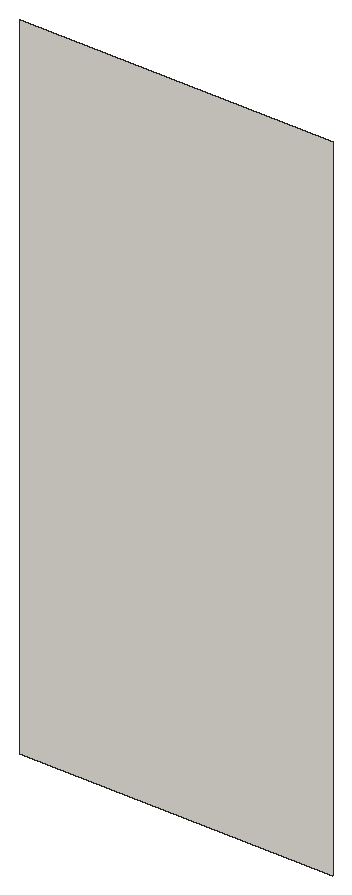
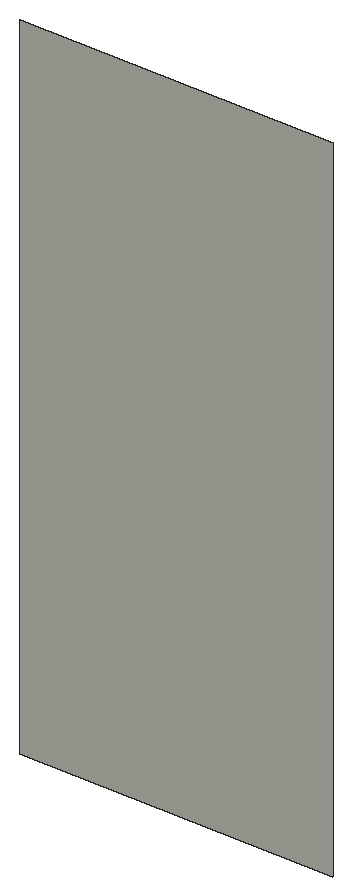
# SketchUp Ruby script. Lengths in inches.
U = 1.inch
M = Sketchup.active_model
def pt(a) = Geom::Point3d.new(a.map { |v| v * U })
def face(e, loops, mat)
  f = e.add_face(loops[0].map { |a| pt(a) })
  loops[1..].each { |l| e.add_face(l.map { |a| pt(a) }).erase! }
  f.material = f.back_material = mat if mat
  f
end
# faces: each face lists its corners as indices into pts; further lists are holes
def faces(e, pts, list, mat = nil) = list.each { |f| face(e, (f[0].is_a?(Array) ? f : [f]).map { |l| l.map { |i| pts[i] } }, mat) }
# xy, xz, yz: faces in a plane at the given z, y or x. An outline is a flat list of corners, or four numbers for a rectangle; further outlines are holes
def ring(l) = l.size == 4 ? [[l[0], l[1]], [l[2], l[1]], [l[2], l[3]], [l[0], l[3]]] : l.each_slice(2).to_a
def flat(e, list, mat, &to3) = list.each { |f| face(e, (f[0].is_a?(Array) ? f : [f]).map { |l| ring(l).map { |u, v| to3.(u, v) } }, mat) }
def xy(e, z, list, mat = nil) = flat(e, list, mat) { |x, y| [x, y, z] }
def xz(e, y, list, mat = nil) = flat(e, list, mat) { |x, z| [x, y, z] }
def yz(e, x, list, mat = nil) = flat(e, list, mat) { |y, z| [x, y, z] }
def lines(e, pts, list) = list.each { |a, b| e.add_line(pt(pts[a]), pt(pts[b])) }
# prism: a flat outline (further loops are holes) pulled along v
def prism(e, loops, v, mat = nil)
  f = face(e, loops, mat); d = Geom::Vector3d.new(v.map { |x| x * U })
  f.pushpull(f.normal.samedirection?(d) ? d.length : -d.length)
end
def box(e, o, s, mat = nil) = prism(e, [[o, [o[0] + s[0], o[1], o[2]], [o[0] + s[0], o[1] + s[1], o[2]], [o[0], o[1] + s[1], o[2]]]], [0, 0, s[2]], mat)
def at(x, y, z, deg = 0) = Geom::Transformation.translation(pt([x, y, z])) * Geom::Transformation.rotation(ORIGIN, Z_AXIS, deg.degrees)
def axes(o, x, y, z) = Geom::Transformation.new([*x, 0, *y, 0, *z, 0, *pt(o).to_a, 1])
def part(name) = M.definitions.add(name)
# library, detail: a bought-in or finely detailed component or shape, given as its bounding box
def library(name, o, s) = part(name).tap { |d| box(d.entities, o, s) }
def detail(e, o, s) = box(e.add_group.entities, o, s)
def put(e, d, t, mat = nil) = e.add_instance(d, t).tap { |i| i.material = mat if mat }
def group(e, t, mat = nil) = e.add_group.tap { |g| g.transformation = t; g.material = mat if mat }.entities
root = M.entities
M.materials.add("[Tile Limestone Large]").color = [237, 234, 224]
xz(root,137.79,[[46.1875,17.625,111.84,155.84]],"[Tile Limestone Large]")
